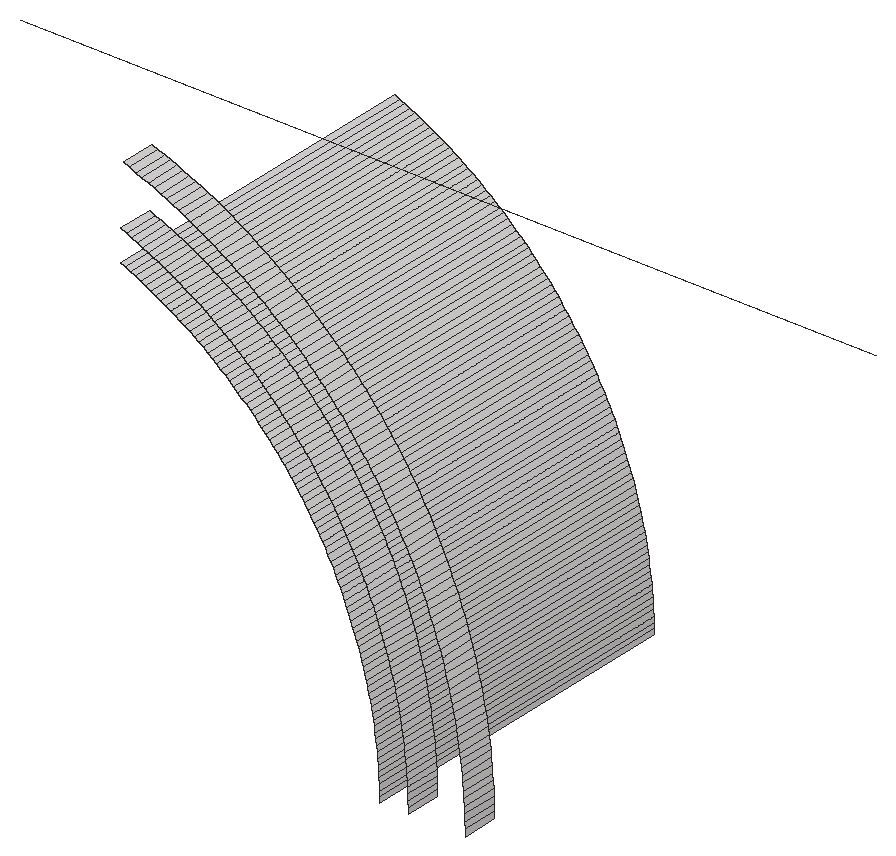
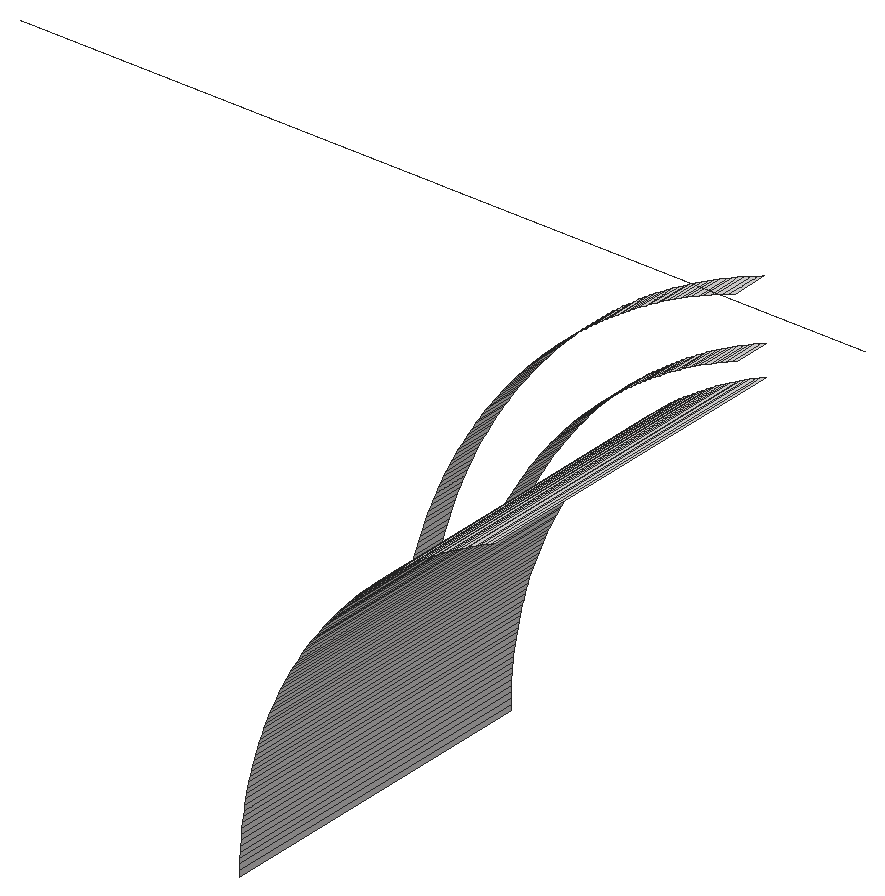
# SketchUp Ruby script. Lengths in inches.
U = 1.inch
M = Sketchup.active_model
def pt(a) = Geom::Point3d.new(a.map { |v| v * U })
def face(e, loops, mat)
  f = e.add_face(loops[0].map { |a| pt(a) })
  loops[1..].each { |l| e.add_face(l.map { |a| pt(a) }).erase! }
  f.material = f.back_material = mat if mat
  f
end
# faces: each face lists its corners as indices into pts; further lists are holes
def faces(e, pts, list, mat = nil) = list.each { |f| face(e, (f[0].is_a?(Array) ? f : [f]).map { |l| l.map { |i| pts[i] } }, mat) }
# xy, xz, yz: faces in a plane at the given z, y or x. An outline is a flat list of corners, or four numbers for a rectangle; further outlines are holes
def ring(l) = l.size == 4 ? [[l[0], l[1]], [l[2], l[1]], [l[2], l[3]], [l[0], l[3]]] : l.each_slice(2).to_a
def flat(e, list, mat, &to3) = list.each { |f| face(e, (f[0].is_a?(Array) ? f : [f]).map { |l| ring(l).map { |u, v| to3.(u, v) } }, mat) }
def xy(e, z, list, mat = nil) = flat(e, list, mat) { |x, y| [x, y, z] }
def xz(e, y, list, mat = nil) = flat(e, list, mat) { |x, z| [x, y, z] }
def yz(e, x, list, mat = nil) = flat(e, list, mat) { |y, z| [x, y, z] }
def lines(e, pts, list) = list.each { |a, b| e.add_line(pt(pts[a]), pt(pts[b])) }
# prism: a flat outline (further loops are holes) pulled along v
def prism(e, loops, v, mat = nil)
  f = face(e, loops, mat); d = Geom::Vector3d.new(v.map { |x| x * U })
  f.pushpull(f.normal.samedirection?(d) ? d.length : -d.length)
end
def box(e, o, s, mat = nil) = prism(e, [[o, [o[0] + s[0], o[1], o[2]], [o[0] + s[0], o[1] + s[1], o[2]], [o[0], o[1] + s[1], o[2]]]], [0, 0, s[2]], mat)
def at(x, y, z, deg = 0) = Geom::Transformation.translation(pt([x, y, z])) * Geom::Transformation.rotation(ORIGIN, Z_AXIS, deg.degrees)
def axes(o, x, y, z) = Geom::Transformation.new([*x, 0, *y, 0, *z, 0, *pt(o).to_a, 1])
def part(name) = M.definitions.add(name)
# library, detail: a bought-in or finely detailed component or shape, given as its bounding box
def library(name, o, s) = part(name).tap { |d| box(d.entities, o, s) }
def detail(e, o, s) = box(e.add_group.entities, o, s)
def put(e, d, t, mat = nil) = e.add_instance(d, t).tap { |i| i.material = mat if mat }
def group(e, t, mat = nil) = e.add_group.tap { |g| g.transformation = t; g.material = mat if mat }.entities
root = M.entities
M.materials.add("[Quartz Light Brown]").color = [215, 212, 212]
yz(root,464.99,[[143,336.39,155,336.59]],"[Quartz Light Brown]")
yz(root,465,[[143,336,155,336.2]],"[Quartz Light Brown]")
yz(root,465.99,[[143,336.42,144.25,336.63]],"[Quartz Light Brown]")
yz(root,466,[[143,336,144.25,336.21]],"[Quartz Light Brown]")
yz(root,467.99,[[143,336.47,144.25,336.71]],"[Quartz Light Brown]")
yz(root,468,[[143,336,144.25,336.24]],"[Quartz Light Brown]")
p = [[465,143,336.2],[464.99,143,336.39],[464.99,155,336.39],[465,155,336.2],[465.99,143,336.42],[466,143,336.21],
  [466,144.25,336.21],[465.99,144.25,336.42],[468,144.25,336.24],[468,143,336.24],[467.99,143,336.47],[467.99,144.25,336.47],
  [464.99,143,336.59],[464.98,143,336.79],[464.98,155,336.79],[464.99,155,336.59],[465.98,143,336.84],[465.99,143,336.63],
  [465.99,144.25,336.63],[465.98,144.25,336.84],[467.99,144.25,336.71],[467.99,143,336.71],[467.98,143,336.94],[467.98,144.25,336.94],
  [464.97,143,336.98],[464.97,155,336.98],[465.97,143,337.05],[465.97,144.25,337.05],[467.96,143,337.18],[467.96,144.25,337.18],
  [464.95,143,337.18],[464.95,155,337.18],[465.95,143,337.26],[465.95,144.25,337.26],[464.9375,143,337.37],[464.9375,155,337.37],
  [467.94,143,337.41],[467.94,144.25,337.41],[465.93,143,337.46],[465.93,144.25,337.46],[464.92,143,337.57],[464.92,155,337.57],
  [467.92,143,337.65],[467.92,144.25,337.65],[465.91,143,337.67],[465.91,144.25,337.67],[464.9,143,337.76],[464.9,155,337.76],
  [467.9,143,337.88],[467.9,144.25,337.88],[465.89,143,337.88],[465.89,144.25,337.88],[464.87,143,337.96],[464.87,155,337.96],
  [465.86,143,338.09],[465.86,144.25,338.09],[467.875,143,338.12],[467.875,144.25,338.12],[464.84,143,338.15],[464.84,155,338.15],
  [465.83,143,338.3],[465.83,144.25,338.3],[467.85,143,338.35],[467.85,144.25,338.35],[464.82,143,338.35],[464.82,155,338.35],
  [464.78,143,338.54],[464.78,155,338.54],[465.8,143,338.5],[465.8,144.25,338.5],[467.8125,143,338.58],[467.8125,144.25,338.58],
  [464.75,143,338.73],[464.75,155,338.73],[465.77,143,338.71],[465.77,144.25,338.71],[467.78,143,338.82],[467.78,144.25,338.82],
  [464.71,143,338.93],[464.71,155,338.93],[465.73,143,338.92],[465.73,144.25,338.92],[467.74,143,339.05],[467.74,144.25,339.05],
  [464.67,143,339.12],[464.67,155,339.12],[465.69,143,339.12],[465.69,144.25,339.12],[467.7,143,339.28],[467.7,144.25,339.28],
  [464.63,143,339.31],[464.63,155,339.31],[465.65,143,339.33],[465.65,144.25,339.33],[464.59,143,339.5],[464.59,155,339.5],
  [465.61,143,339.53],[465.61,144.25,339.53],[467.65,143,339.51],[467.65,144.25,339.51],[464.54,143,339.69],[464.54,155,339.69],
  [465.56,143,339.74],[465.56,144.25,339.74],[467.61,143,339.74],[467.61,144.25,339.74],[464.49,143,339.88],[464.49,155,339.88],
  [465.51,143,339.9375],[465.51,144.25,339.9375],[467.56,143,339.97],[467.56,144.25,339.97],[464.4375,143,340.07],[464.4375,155,340.07],
  [465.45,143,340.14],[465.45,144.25,340.14],[467.5,143,340.2],[467.5,144.25,340.2],[464.38,143,340.26],[464.38,155,340.26],
  [465.4,143,340.34],[465.4,144.25,340.34],[467.45,143,340.43],[467.45,144.25,340.43],[464.33,143,340.45],[464.33,155,340.45],
  [465.34,143,340.54],[465.34,144.25,340.54],[464.27,143,340.64],[464.27,155,340.64],[467.39,143,340.66],[467.39,144.25,340.66],
  [465.28,143,340.74],[465.28,144.25,340.74],[464.2,143,340.82],[464.2,155,340.82],[465.22,143,340.94],[465.22,144.25,340.94],
  [467.32,143,340.89],[467.32,144.25,340.89],[464.14,143,341.01],[464.14,155,341.01],[465.15,143,341.14],[465.15,144.25,341.14],
  [467.26,143,341.11],[467.26,144.25,341.11],[464.07,143,341.19],[464.07,155,341.19],[465.08,143,341.34],[465.08,144.25,341.34],
  [467.19,143,341.34],[467.19,144.25,341.34],[464,143,341.375],[464,155,341.375],[465.01,143,341.54],[465.01,144.25,341.54],
  [467.12,143,341.5625],[467.12,144.25,341.5625],[463.93,143,341.56],[463.93,155,341.56],[464.9375,143,341.73],[464.9375,144.25,341.73],
  [463.86,143,341.74],[463.86,155,341.74],[467.04,143,341.79],[467.04,144.25,341.79],[463.78,143,341.92],[463.78,155,341.92],
  [464.86,143,341.93],[464.86,144.25,341.93],[466.97,143,342.01],[466.97,144.25,342.01],[463.7,143,342.1],[463.7,155,342.1],
  [464.78,143,342.12],[464.78,144.25,342.12],[466.89,143,342.23],[466.89,144.25,342.23],[463.62,143,342.28],[463.62,155,342.28],
  [464.7,143,342.32],[464.7,144.25,342.32],[466.8,143,342.45],[466.8,144.25,342.45],[463.54,143,342.46],[463.54,155,342.46],
  [464.62,143,342.51],[464.62,144.25,342.51],[463.45,143,342.63],[463.45,155,342.63],[464.53,143,342.7],[464.53,144.25,342.7],
  [466.72,143,342.67],[466.72,144.25,342.67],[463.37,143,342.81],[463.37,155,342.81],[464.44,143,342.89],[464.44,144.25,342.89],
  [466.63,143,342.89],[466.63,144.25,342.89],[463.27,143,342.98],[463.27,155,342.98],[464.35,143,343.08],[464.35,144.25,343.08],
  [466.54,143,343.11],[466.54,144.25,343.11],[463.18,143,343.16],[463.18,155,343.16],[464.26,143,343.26],[464.26,144.25,343.26],
  [466.44,143,343.32],[466.44,144.25,343.32],[463.09,143,343.33],[463.09,155,343.33],[462.99,143,343.5],[462.99,155,343.5],
  [464.16,143,343.45],[464.16,144.25,343.45],[466.35,143,343.54],[466.35,144.25,343.54],[464.0625,143,343.63],[464.0625,144.25,343.63],
  [462.89,143,343.67],[462.89,155,343.67],[466.25,143,343.75],[466.25,144.25,343.75],[463.96,143,343.82],[463.96,144.25,343.82],
  [462.79,143,343.84],[462.79,155,343.84],[466.14,143,343.96],[466.14,144.25,343.96],[462.6875,143,344],[462.6875,155,344],
  [463.86,143,344],[463.86,144.25,344],[462.58,143,344.17],[462.58,155,344.17],[463.75,143,344.18],[463.75,144.25,344.18],
  [466.04,143,344.17],[466.04,144.25,344.17],[462.47,143,344.33],[462.47,155,344.33],[463.64,143,344.36],[463.64,144.25,344.36],
  [465.93,143,344.38],[465.93,144.25,344.38],[462.36,143,344.5],[462.36,155,344.5],[463.53,143,344.54],[463.53,144.25,344.54],
  [465.82,143,344.59],[465.82,144.25,344.59],[462.25,143,344.66],[462.25,155,344.66],[463.42,143,344.71],[463.42,144.25,344.71],
  [465.7,143,344.8],[465.7,144.25,344.8],[462.14,143,344.82],[462.14,155,344.82],[463.3,143,344.89],[463.3,144.25,344.89],
  [462.02,143,344.97],[462.02,155,344.97],[465.59,143,345],[465.59,144.25,345],[463.1875,143,345.0625],[463.1875,144.25,345.0625],
  [461.9,143,345.13],[461.9,155,345.13],[465.47,143,345.2],[465.47,144.25,345.2],[461.78,143,345.29],[461.78,155,345.29],
  [463.07,143,345.23],[463.07,144.25,345.23],[462.94,143,345.4],[462.94,144.25,345.4],[465.35,143,345.4],[465.35,144.25,345.4],
  [461.66,143,345.44],[461.66,155,345.44],[461.53,143,345.59],[461.53,155,345.59],[462.82,143,345.57],[462.82,144.25,345.57],
  [465.22,143,345.61],[465.22,144.25,345.61],[461.41,143,345.74],[461.41,155,345.74],[462.69,143,345.74],[462.69,144.25,345.74],
  [465.1,143,345.8],[465.1,144.25,345.8],[461.28,143,345.89],[461.28,155,345.89],[462.57,143,345.91],[462.57,144.25,345.91],
  [464.97,143,346],[464.97,144.25,346],[461.15,143,346.04],[461.15,155,346.04],[462.43,143,346.07],[462.43,144.25,346.07],
  [461.01,143,346.18],[461.01,155,346.18],[464.83,143,346.2],[464.83,144.25,346.2],[462.3,143,346.23],[462.3,144.25,346.23],
  [460.88,143,346.33],[460.88,155,346.33],[462.17,143,346.39],[462.17,144.25,346.39],[464.7,143,346.39],[464.7,144.25,346.39],
  [460.74,143,346.47],[460.74,155,346.47],[462.03,143,346.55],[462.03,144.25,346.55],[464.5625,143,346.58],[464.5625,144.25,346.58],
  [460.61,143,346.61],[460.61,155,346.61],[461.89,143,346.71],[461.89,144.25,346.71],[460.47,143,346.74],[460.47,155,346.74],
  [464.42,143,346.77],[464.42,144.25,346.77],[460.33,143,346.88],[460.33,155,346.88],[461.75,143,346.86],[461.75,144.25,346.86],
  [464.28,143,346.96],[464.28,144.25,346.96],[460.18,143,347.01],[460.18,155,347.01],[461.61,143,347.01],[461.61,144.25,347.01],
  [460.04,143,347.15],[460.04,155,347.15],[461.46,143,347.16],[461.46,144.25,347.16],[464.14,143,347.14],[464.14,144.25,347.14],
  [459.89,143,347.28],[459.89,155,347.28],[463.99,143,347.33],[463.99,144.25,347.33],[461.3125,143,347.3125],[461.3125,144.25,347.3125],
  [459.74,143,347.41],[459.74,155,347.41],[461.16,143,347.46],[461.16,144.25,347.46],[463.84,143,347.51],[463.84,144.25,347.51],
  [459.59,143,347.53],[459.59,155,347.53],[459.44,143,347.66],[459.44,155,347.66],[461.01,143,347.61],[461.01,144.25,347.61],
  [463.6875,143,347.69],[463.6875,144.25,347.69],[460.86,143,347.75],[460.86,144.25,347.75],[459.29,143,347.78],[459.29,155,347.78],
  [460.71,143,347.89],[460.71,144.25,347.89],[463.53,143,347.87],[463.53,144.25,347.87],[459.13,143,347.9],[459.13,155,347.9],
  [458.97,143,348.02],[458.97,155,348.02],[460.55,143,348.03],[460.55,144.25,348.03],[463.375,143,348.04],[463.375,144.25,348.04],
  [458.82,143,348.14],[458.82,155,348.14],[460.39,143,348.17],[460.39,144.25,348.17],[463.22,143,348.22],[463.22,144.25,348.22],
  [458.66,143,348.25],[458.66,155,348.25],[458.5,143,348.36],[458.5,155,348.36],[460.23,143,348.3],[460.23,144.25,348.3],
  [463.06,143,348.39],[463.06,144.25,348.39],[460.07,143,348.43],[460.07,144.25,348.43],[458.33,143,348.47],[458.33,155,348.47],
  [459.91,143,348.57],[459.91,144.25,348.57],[462.89,143,348.56],[462.89,144.25,348.56],[458.17,143,348.58],[458.17,155,348.58],
  [458,143,348.6875],[458,155,348.6875],[459.74,143,348.69],[459.74,144.25,348.69],[462.73,143,348.73],[462.73,144.25,348.73],
  [457.84,143,348.79],[457.84,155,348.79],[459.57,143,348.82],[459.57,144.25,348.82],[462.56,143,348.89],[462.56,144.25,348.89],
  [457.67,143,348.89],[457.67,155,348.89],[459.4,143,348.94],[459.4,144.25,348.94],[457.5,143,348.99],[457.5,155,348.99],
  [459.23,143,349.07],[459.23,144.25,349.07],[462.39,143,349.06],[462.39,144.25,349.06],[457.33,143,349.09],[457.33,155,349.09],
  [457.16,143,349.18],[457.16,155,349.18],[459.0625,143,349.1875],[459.0625,144.25,349.1875],[462.22,143,349.22],[462.22,144.25,349.22],
  [456.98,143,349.27],[456.98,155,349.27],[458.89,143,349.3],[458.89,144.25,349.3],[462.04,143,349.375],[462.04,144.25,349.375],
  [456.81,143,349.37],[456.81,155,349.37],[458.71,143,349.42],[458.71,144.25,349.42],[456.63,143,349.45],[456.63,155,349.45],
  [458.54,143,349.53],[458.54,144.25,349.53],[461.87,143,349.53],[461.87,144.25,349.53],[456.46,143,349.54],[456.28,143,349.62],
  [456.28,155,349.62],[456.46,155,349.54],[458.36,143,349.64],[458.36,144.25,349.64],[461.69,143,349.6875],[461.69,144.25,349.6875],
  [456.1,143,349.7],[456.1,155,349.7],[458.18,143,349.75],[458.18,144.25,349.75],[455.92,143,349.78],[455.92,155,349.78],
  [461.51,143,349.84],[461.51,144.25,349.84],[458,143,349.86],[458,144.25,349.86],[461.33,143,349.99],[461.33,144.25,349.99],
  [457.82,143,349.96],[457.82,144.25,349.96],[457.63,143,350.0625],[457.63,144.25,350.0625],[461.14,143,350.14],[461.14,144.25,350.14],
  [457.45,143,350.16],[457.45,144.25,350.16],[460.96,143,350.28],[460.96,144.25,350.28],[457.26,143,350.26],[457.26,144.25,350.26],
  [456.89,143,350.44],[457.08,143,350.35],[457.08,144.25,350.35],[456.89,144.25,350.44],[460.77,143,350.42],[460.77,144.25,350.42],
  [456.7,143,350.53],[456.7,144.25,350.53],[460.58,143,350.5625],[460.58,144.25,350.5625],[456.51,143,350.62],[456.51,144.25,350.62],
  [456.32,143,350.7],[456.32,144.25,350.7],[460.39,143,350.7],[460.39,144.25,350.7],[456.12,143,350.78],[456.12,144.25,350.78],
  [460.2,143,350.83],[460.2,144.25,350.83],[455.93,143,350.86],[455.93,144.25,350.86],[460,143,350.97],[460,144.25,350.97],
  [459.8,143,351.1],[459.8,144.25,351.1],[459.61,143,351.22],[459.61,144.25,351.22],[459.4,143,351.35],[459.4,144.25,351.35],
  [459.2,143,351.47],[459.2,144.25,351.47],[459,143,351.59],[459,144.25,351.59],[458.8,143,351.7],[458.8,144.25,351.7],
  [458.59,143,351.82],[458.59,144.25,351.82],[458.38,143,351.93],[458.38,144.25,351.93],[458.17,143,352.04],[458.17,144.25,352.04],
  [457.96,143,352.14],[457.96,144.25,352.14],[457.75,143,352.25],[457.75,144.25,352.25],[457.54,143,352.35],[457.54,144.25,352.35],
  [457.32,143,352.44],[457.32,144.25,352.44],[457.11,143,352.54],[457.11,144.25,352.54],[456.89,143,352.63],[456.89,144.25,352.63],
  [456.67,143,352.72],[456.67,144.25,352.72],[456.45,143,352.8],[456.45,144.25,352.8],[456.23,143,352.89],[456.23,144.25,352.89],
  [456.01,143,352.97],[456.01,144.25,352.97],[450,146,354],[480,146,354]]
faces(root,p,[[0,1,2,3],[4,5,6,7],[8,9,10,11],[12,13,14,15],[16,17,18,19],[20,21,22,23],[13,24,25,14],[26,16,19,27],
  [23,22,28,29],[24,30,31,25],[32,26,27,33],[30,34,35,31],[29,28,36,37],[38,32,33,39],[34,40,41,35],[37,36,42,43],
  [44,38,39,45],[40,46,47,41],[43,42,48,49],[50,44,45,51],[46,52,53,47],[54,50,51,55],[49,48,56,57],[52,58,59,53],
  [60,54,55,61],[57,56,62,63],[58,64,65,59],[64,66,67,65],[68,60,61,69],[63,62,70,71],[66,72,73,67],[74,68,69,75],
  [71,70,76,77],[72,78,79,73],[80,74,75,81],[77,76,82,83],[78,84,85,79],[86,80,81,87],[83,82,88,89],[84,90,91,85],
  [92,86,87,93],[90,94,95,91],[96,92,93,97],[89,88,98,99],[94,100,101,95],[102,96,97,103],[99,98,104,105],[100,106,107,101],
  [108,102,103,109],[105,104,110,111],[106,112,113,107],[114,108,109,115],[111,110,116,117],[112,118,119,113],[120,114,115,121],[117,116,122,123],
  [118,124,125,119],[126,120,121,127],[124,128,129,125],[123,122,130,131],[132,126,127,133],[128,134,135,129],[136,132,133,137],[131,130,138,139],
  [134,140,141,135],[142,136,137,143],[139,138,144,145],[140,146,147,141],[148,142,143,149],[145,144,150,151],[146,152,153,147],[154,148,149,155],
  [151,150,156,157],[152,158,159,153],[160,154,155,161],[158,162,163,159],[157,156,164,165],[162,166,167,163],[168,160,161,169],[165,164,170,171],
  [166,172,173,167],[174,168,169,175],[171,170,176,177],[172,178,179,173],[180,174,175,181],[177,176,182,183],[178,184,185,179],[186,180,181,187],
  [184,188,189,185],[190,186,187,191],[183,182,192,193],[188,194,195,189],[196,190,191,197],[193,192,198,199],[194,200,201,195],[202,196,197,203],
  [199,198,204,205],[200,206,207,201],[208,202,203,209],[205,204,210,211],[206,212,213,207],[212,214,215,213],[216,208,209,217],[211,210,218,219],
  [220,216,217,221],[214,222,223,215],[219,218,224,225],[226,220,221,227],[222,228,229,223],[225,224,230,231],[228,232,233,229],[234,226,227,235],
  [232,236,237,233],[238,234,235,239],[231,230,240,241],[236,242,243,237],[244,238,239,245],[241,240,246,247],[242,248,249,243],[250,244,245,251],
  [247,246,252,253],[248,254,255,249],[256,250,251,257],[253,252,258,259],[254,260,261,255],[262,256,257,263],[260,264,265,261],[259,258,266,267],
  [268,262,263,269],[264,270,271,265],[267,266,272,273],[270,274,275,271],[276,268,269,277],[278,276,277,279],[273,272,280,281],[274,282,283,275],
  [282,284,285,283],[286,278,279,287],[281,280,288,289],[284,290,291,285],[292,286,287,293],[289,288,294,295],[290,296,297,291],[298,292,293,299],
  [295,294,300,301],[296,302,303,297],[304,298,299,305],[302,306,307,303],[301,300,308,309],[310,304,305,311],[306,312,313,307],[314,310,311,315],
  [309,308,316,317],[312,318,319,313],[320,314,315,321],[317,316,322,323],[318,324,325,319],[326,320,321,327],[324,328,329,325],[323,322,330,331],
  [328,332,333,329],[334,326,327,335],[331,330,336,337],[332,338,339,333],[340,334,335,341],[338,342,343,339],[344,340,341,345],[337,336,346,347],
  [342,348,349,343],[347,346,350,351],[352,344,345,353],[348,354,355,349],[356,352,353,357],[351,350,358,359],[354,360,361,355],[360,362,363,361],
  [364,356,357,365],[359,358,366,367],[368,364,365,369],[362,370,371,363],[372,368,369,373],[367,366,374,375],[370,376,377,371],[376,378,379,377],
  [380,372,373,381],[375,374,382,383],[378,384,385,379],[386,380,381,387],[383,382,388,389],[384,390,391,385],[390,392,393,391],[394,386,387,395],
  [389,388,396,397],[398,394,395,399],[392,400,401,393],[402,398,399,403],[397,396,404,405],[400,406,407,401],[406,408,409,407],[410,402,403,411],
  [405,404,412,413],[408,414,415,409],[416,410,411,417],[413,412,418,419],[414,420,421,415],[422,416,417,423],[420,424,425,421],[426,422,423,427],
  [419,418,428,429],[424,430,431,425],[430,432,433,431],[434,426,427,435],[429,428,436,437],[432,438,439,433],[440,434,435,441],[437,436,442,443],
  [438,444,445,439],[446,440,441,447],[444,448,449,445],[450,446,447,451],[443,442,452,453],[454,455,456,457],[448,454,457,449],[458,450,451,459],
  [453,452,460,461],[455,462,463,456],[464,458,459,465],[462,466,467,463],[461,460,468,469],[470,464,465,471],[469,468,472,473],[474,470,471,475],
  [476,474,475,477],[473,472,478,479],[480,476,477,481],[479,478,482,483],[484,480,481,485],[486,487,488,489],[487,484,485,488],[483,482,490,491],
  [492,486,489,493],[491,490,494,495],[496,492,493,497],[498,496,497,499],[495,494,500,501],[502,498,499,503],[501,500,504,505],[506,502,503,507],
  [505,504,508,509],[509,508,510,511],[511,510,512,513],[513,512,514,515],[515,514,516,517],[517,516,518,519],[519,518,520,521],[521,520,522,523],
  [523,522,524,525],[525,524,526,527],[527,526,528,529],[529,528,530,531],[531,530,532,533],[533,532,534,535],[535,534,536,537],[537,536,538,539],
  [539,538,540,541],[541,540,542,543],[543,542,544,545],[545,544,546,547]],"[Quartz Light Brown]")
lines(root,p,[[548,549]])
